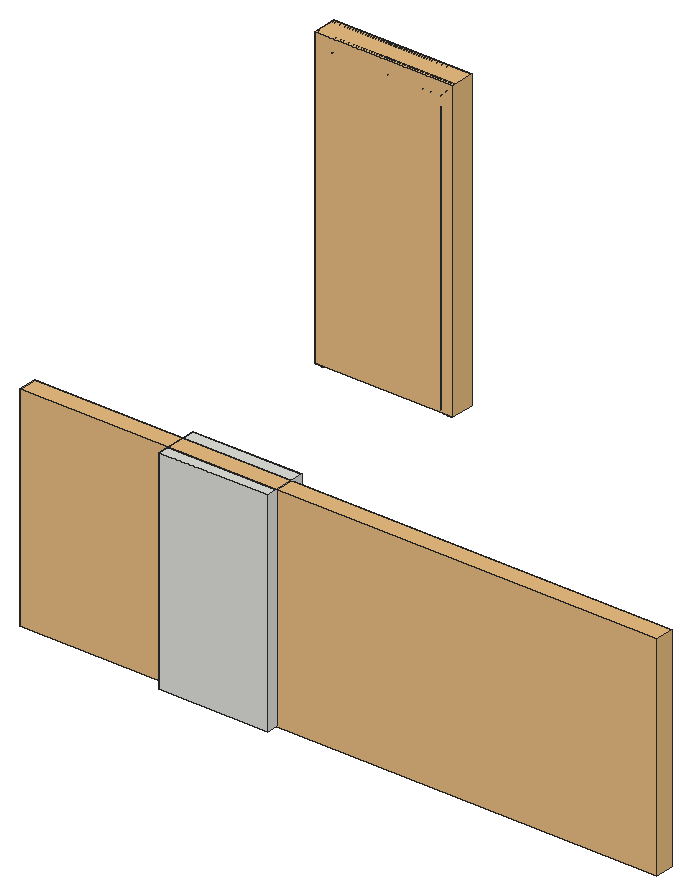
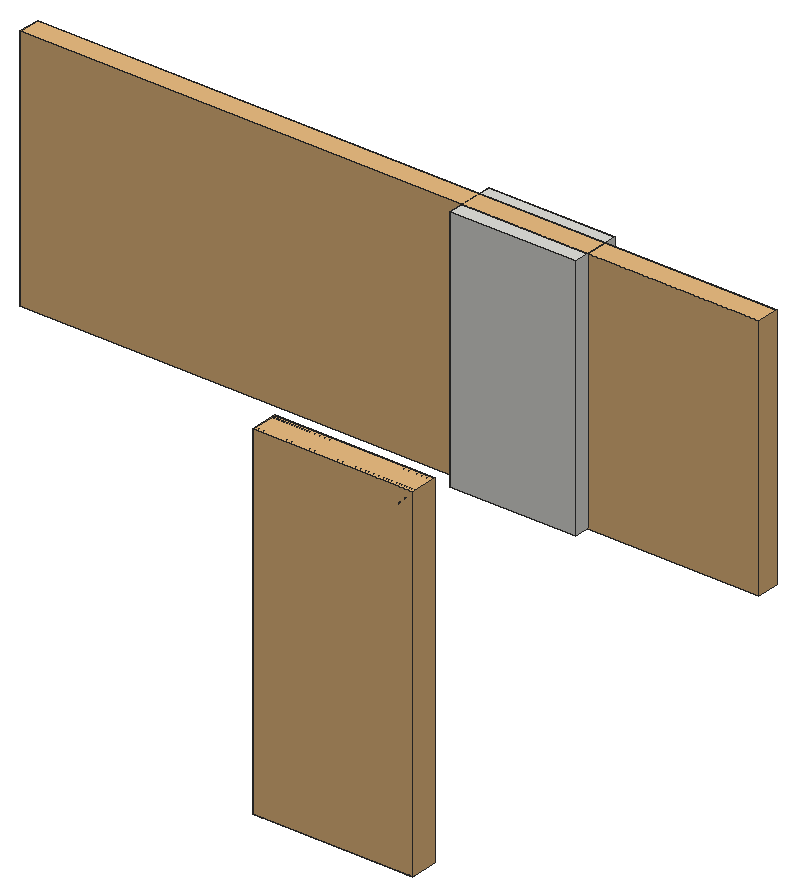
# SketchUp Ruby script. Lengths in inches.
U = 1.inch
M = Sketchup.active_model
def pt(a) = Geom::Point3d.new(a.map { |v| v * U })
def face(e, loops, mat)
  f = e.add_face(loops[0].map { |a| pt(a) })
  loops[1..].each { |l| e.add_face(l.map { |a| pt(a) }).erase! }
  f.material = f.back_material = mat if mat
  f
end
# faces: each face lists its corners as indices into pts; further lists are holes
def faces(e, pts, list, mat = nil) = list.each { |f| face(e, (f[0].is_a?(Array) ? f : [f]).map { |l| l.map { |i| pts[i] } }, mat) }
# xy, xz, yz: faces in a plane at the given z, y or x. An outline is a flat list of corners, or four numbers for a rectangle; further outlines are holes
def ring(l) = l.size == 4 ? [[l[0], l[1]], [l[2], l[1]], [l[2], l[3]], [l[0], l[3]]] : l.each_slice(2).to_a
def flat(e, list, mat, &to3) = list.each { |f| face(e, (f[0].is_a?(Array) ? f : [f]).map { |l| ring(l).map { |u, v| to3.(u, v) } }, mat) }
def xy(e, z, list, mat = nil) = flat(e, list, mat) { |x, y| [x, y, z] }
def xz(e, y, list, mat = nil) = flat(e, list, mat) { |x, z| [x, y, z] }
def yz(e, x, list, mat = nil) = flat(e, list, mat) { |y, z| [x, y, z] }
def lines(e, pts, list) = list.each { |a, b| e.add_line(pt(pts[a]), pt(pts[b])) }
# prism: a flat outline (further loops are holes) pulled along v
def prism(e, loops, v, mat = nil)
  f = face(e, loops, mat); d = Geom::Vector3d.new(v.map { |x| x * U })
  f.pushpull(f.normal.samedirection?(d) ? d.length : -d.length)
end
def box(e, o, s, mat = nil) = prism(e, [[o, [o[0] + s[0], o[1], o[2]], [o[0] + s[0], o[1] + s[1], o[2]], [o[0], o[1] + s[1], o[2]]]], [0, 0, s[2]], mat)
def at(x, y, z, deg = 0) = Geom::Transformation.translation(pt([x, y, z])) * Geom::Transformation.rotation(ORIGIN, Z_AXIS, deg.degrees)
def axes(o, x, y, z) = Geom::Transformation.new([*x, 0, *y, 0, *z, 0, *pt(o).to_a, 1])
def part(name) = M.definitions.add(name)
# library, detail: a bought-in or finely detailed component or shape, given as its bounding box
def library(name, o, s) = part(name).tap { |d| box(d.entities, o, s) }
def detail(e, o, s) = box(e.add_group.entities, o, s)
def put(e, d, t, mat = nil) = e.add_instance(d, t).tap { |i| i.material = mat if mat }
def group(e, t, mat = nil) = e.add_group.tap { |g| g.transformation = t; g.material = mat if mat }.entities
root = M.entities
M.materials.add("Material \#0").color = [86, 53, 35]
M.materials.add("Material \#1").color = [140, 140, 140]
c1 = library("Entrance gate assembly",[-0.09,68.76,-0.1],[180.01,5.32,60.06])
c2 = part("3DGeom~20_Defintion")
xy(c2.entities,0,[[-976.3,-241.71,-976.3,-223.46,23.7,-241.71],[23.7,-241.71,-976.3,-223.46,5.45,-223.46],[23.7,-241.71,5.45,-223.46,5.45,0],[23.7,-241.71,5.45,0,23.7,0],[-976.3,-223.46,-976.3,-211.85,5.45,-223.46],
  [5.45,-223.46,-976.3,-211.85,-6.16,-211.85],[5.45,-223.46,-6.16,-211.85,-6.16,0],[5.45,-223.46,-6.16,0,5.45,0],[-6.16,0,-6.16,211.85,5.45,223.46],[-6.16,0,5.45,223.46,5.45,0],
  [5.45,0,23.7,241.71,23.7,0],[5.45,0,5.45,223.46,23.7,241.71],[-976.3,211.85,-976.3,223.46,5.45,223.46],[-976.3,211.85,5.45,223.46,-6.16,211.85],[-976.3,223.46,-976.3,241.71,23.7,241.71],
  [-976.3,223.46,23.7,241.71,5.45,223.46]],"Material \#0")
c3 = part("3DGeom~18_Defintion")
xz(c3.entities,-241.71,[[-976.3,0,23.7,0,23.7,7.58],[-976.3,0,23.7,7.58,-976.3,7.58]],"Material \#0")
xz(c3.entities,241.71,[[-976.3,0,-976.3,7.58,23.7,7.58],[-976.3,0,23.7,7.58,23.7,0]],"Material \#0")
yz(c3.entities,23.7,[[-241.71,0,0,0,-241.71,7.58],[0,0,0,7.58,-241.71,7.58],[0,0,241.71,0,241.71,7.58],[0,0,241.71,7.58,0,7.58]],"Material \#0")
c4 = part("3DGeom~17_Defintion")
yz(c4.entities,-1908.8,[[-436.03,-21.87,-436.73,-21.5,-435.91,-21.83],[436.03,-21.87,435.91,-21.83,436.73,-21.5],[-435.91,-21.83,-436.73,-21.5,-436.15,-21.125],[-435.91,-21.83,-436.15,-21.125,-435.87,-21.72],[435.91,-21.83,435.87,-21.72,436.15,-21.125],
  [435.91,-21.83,436.15,-21.125,436.73,-21.5],[-436.73,-21.5,-484.73,-21.37,-436.15,-1.11],[-471.46,-21.5,-484.73,-21.37,-436.73,-21.5],[-477.2,-21.5,-484.73,-21.37,-471.46,-21.5],[-481.82,-21.5,-484.73,-21.37,-477.2,-21.5],
  [-436.73,-21.5,-436.15,-1.11,-436.15,-21.125],[436.73,-21.5,436.15,-21.125,471.46,-21.5],[471.46,-21.5,436.15,-21.125,477.2,-21.5],[477.2,-21.5,436.15,-21.125,499.98,-0.85],[477.2,-21.5,499.98,-0.85,481.82,-21.5],
  [481.82,-21.5,487.35,-21,484.73,-21.37],[481.82,-21.5,491.8,-19.52,487.35,-21],[481.82,-21.5,497.64,-13.67,491.8,-19.52],[481.82,-21.5,499.98,-0.85,497.64,-13.67],[-484.73,-21.37,-498.5,-11.58,-499.84,-0.37],
  [-484.73,-21.37,-499.84,-0.37,-499.4,-0.5],[-484.73,-21.37,-499.4,-0.5,-436.15,-1.11],[-484.73,-21.37,-493.63,-18.42,-498.5,-11.58],[-484.73,-21.37,-489.71,-20.375,-493.63,-18.42],[-484.73,-21.37,-487.35,-21,-489.71,-20.375],
  [436.15,-21.125,436.15,-1.11,436.73,-0.74],[436.15,-21.125,436.73,-0.74,499.98,-0.85],[487.35,-21,491.8,-19.52,489.71,-20.375],[-489.71,-20.375,-491.8,-19.52,-493.63,-18.42],[491.8,-19.52,495.21,-17.08,493.63,-18.42],
  [491.8,-19.52,497.64,-13.67,495.21,-17.08],[-493.63,-18.42,-496.54,-15.5,-498.5,-11.58],[-493.63,-18.42,-495.21,-17.08,-496.54,-15.5],[495.21,-17.08,497.64,-13.67,496.54,-15.5],[-496.54,-15.5,-497.64,-13.67,-498.5,-11.58],
  [497.64,-13.67,499.125,-9.22,498.5,-11.58],[497.64,-13.67,499.625,-3.69,499.125,-9.22],[497.64,-13.67,499.98,-0.85,499.625,-3.69],[-498.5,-11.58,-499.625,-3.69,-499.84,-0.37],[-498.5,-11.58,-499.5,-6.6,-499.625,-3.69],
  [-498.5,-11.58,-499.125,-9.22,-499.5,-6.6],[499.125,-9.22,499.625,-3.69,499.5,-6.6],[-499.625,-3.69,-499.98,-0.85,-500,-0.52],[-499.625,-3.69,-500,-0.52,-499.84,-0.37],[-436.15,-1.11,-499.4,-0.5,-471.46,-0.74],
  [-436.15,-1.11,-471.46,-0.74,-436.73,-0.74],[-436.15,-1.11,-436.73,-0.74,-435.91,-0.41],[-436.15,-1.11,-435.91,-0.41,-435.87,-0.52],[436.15,-1.11,435.87,-0.52,435.91,-0.41],[436.15,-1.11,435.91,-0.41,436.73,-0.74],
  [499.98,-0.85,436.73,-0.74,471.46,-0.74],[499.98,-0.85,471.46,-0.74,499.4,-0.5],[499.98,-0.85,499.4,-0.5,499.96,-0.41],[499.98,-0.85,499.96,-0.41,500,-0.52],[-436.73,-0.74,-436.03,-0.37,-435.91,-0.41],
  [436.73,-0.74,435.91,-0.41,436.03,-0.37],[-500,-0.52,-499.96,-0.41,-499.84,-0.37],[499.4,-0.5,499.84,-0.37,499.96,-0.41],[-499.84,141.21,-499.96,141.25,-499.4,141.35],[-436.03,141.21,-436.73,141.59,-435.91,141.25],
  [436.03,141.21,435.91,141.25,436.73,141.59],[499.84,141.21,484.73,162.21,498.5,152.42],[499.84,141.21,499.4,141.35,484.73,162.21],[499.84,141.21,498.5,152.42,499.625,144.53],[499.84,141.21,499.625,144.53,500,141.37],
  [499.84,141.21,500,141.37,499.96,141.25],[-499.96,141.25,-500,141.37,-499.98,141.69],[-499.96,141.25,-499.98,141.69,-499.4,141.35],[-435.91,141.25,-436.73,141.59,-436.15,141.96],[-435.91,141.25,-436.15,141.96,-435.87,141.37],
  [435.91,141.25,435.87,141.37,436.15,141.96],[435.91,141.25,436.15,141.96,436.73,141.59],[-499.4,141.35,-499.98,141.69,-471.46,141.59],[499.4,141.35,436.15,141.96,484.73,162.21],[499.4,141.35,471.46,141.59,436.15,141.96],
  [500,141.37,499.625,144.53,499.98,141.69],[-436.73,141.59,-499.98,141.69,-436.15,161.97],[-471.46,141.59,-499.98,141.69,-436.73,141.59],[-436.73,141.59,-436.15,161.97,-436.15,141.96],[436.73,141.59,436.15,141.96,471.46,141.59],
  [-499.98,141.69,-477.2,162.34,-436.15,161.97],[-499.98,141.69,-481.82,162.34,-477.2,162.34],[-499.98,141.69,-497.64,154.51,-481.82,162.34],[-499.98,141.69,-499.625,144.53,-497.64,154.51],[436.15,141.96,436.15,161.97,436.73,162.34],
  [436.15,141.96,436.73,162.34,484.73,162.21],[-499.625,144.53,-499.125,150.07,-497.64,154.51],[-499.625,144.53,-499.5,147.44,-499.125,150.07],[499.625,144.53,498.5,152.42,499.5,147.44],[499.5,147.44,498.5,152.42,499.125,150.07],
  [-499.125,150.07,-498.5,152.42,-497.64,154.51],[498.5,152.42,484.73,162.21,493.63,159.26],[498.5,152.42,493.63,159.26,496.54,156.34],[498.5,152.42,496.54,156.34,497.64,154.51],[-497.64,154.51,-491.8,160.36,-481.82,162.34],
  [-497.64,154.51,-495.21,157.92,-491.8,160.36],[-497.64,154.51,-496.54,156.34,-495.21,157.92],[496.54,156.34,493.63,159.26,495.21,157.92],[-495.21,157.92,-493.63,159.26,-491.8,160.36],[493.63,159.26,484.73,162.21,489.71,161.22],
  [493.63,159.26,489.71,161.22,491.8,160.36],[-491.8,160.36,-487.35,161.84,-481.82,162.34],[-491.8,160.36,-489.71,161.22,-487.35,161.84],[489.71,161.22,484.73,162.21,487.35,161.84],[-487.35,161.84,-484.73,162.21,-481.82,162.34],
  [-436.15,161.97,-477.2,162.34,-471.46,162.34],[-436.15,161.97,-471.46,162.34,-436.73,162.34],[-436.15,161.97,-436.73,162.34,-435.91,162.68],[-436.15,161.97,-435.91,162.68,-435.87,162.56],[436.15,161.97,435.87,162.56,435.91,162.68],
  [436.15,161.97,435.91,162.68,436.73,162.34],[484.73,162.21,436.73,162.34,471.46,162.34],[484.73,162.21,471.46,162.34,477.2,162.34],[484.73,162.21,477.2,162.34,481.82,162.34],[-436.73,162.34,-436.03,162.72,-435.91,162.68],
  [436.73,162.34,435.91,162.68,436.03,162.72]],"Material \#0")
c5 = library("3DGeom~16_Defintion",[-962.62,-252.34,-11.22],[1000,504.68,93.46])
c6 = part("3DGeom~22_Defintion")
xz(c6.entities,-210.625,[[-1016.13,2.47,-1016.13,9.96,-16.28,2.47],[-16.28,2.47,-1016.13,9.96,-16.28,9.96],[-1016.13,9.96,-1016.13,51.7,-16.28,51.7],[-1016.13,9.96,-16.28,51.7,-16.28,9.96],[-1016.13,51.7,-1016.13,72.71,-16.28,51.7]],"Material \#0")
xz(c6.entities,210.625,[[-1016.13,2.47,-16.28,2.47,-1016.13,9.96],[-16.28,2.47,-16.28,9.96,-1016.13,9.96],[-1016.13,9.96,-16.28,51.7,-1016.13,51.7],[-1016.13,9.96,-16.28,9.96,-16.28,51.7],[-1016.13,51.7,-16.28,51.7,-1016.13,72.71]],"Material \#0")
yz(c6.entities,-16.28,[[-210.625,2.47,-210.625,9.96,0,9.96],[-210.625,2.47,0,9.96,0,2.47],[0,2.47,0,9.96,210.625,2.47],[210.625,2.47,0,9.96,210.625,9.96],[-210.625,9.96,-210.625,51.7,0,51.7],
  [-210.625,9.96,0,51.7,0,9.96],[0,9.96,0,51.7,210.625,9.96],[210.625,9.96,0,51.7,210.625,51.7],[-210.625,51.7,0,72.71,0,51.7],[0,51.7,0,72.71,210.625,51.7]],"Material \#0")
p = [[-1016.13,-210.625,72.71],[-16.13,-210.77,73.09],[-16.28,-210.625,51.7],[-16.28,-210.625,51.7],[-16.13,-210.77,73.09],[-16.28,0,72.71],
  [-16.13,210.77,73.09],[-16.28,210.625,51.7],[-16.28,210.625,51.7],[-16.13,210.77,73.09],[-1016.13,210.625,72.71]]
faces(c6.entities,p,[[0,1,2],[3,4,5],[5,6,7],[8,9,10]],"Material \#0")
c7 = part("3DGeom~15_Defintion")
xy(c7.entities,0,[[-961.58,-251.9,-958.5,-248.8125,-961.58,-237.8],[-961.58,-251.9,28.8,-248.8125,-958.5,-248.8125],[-961.58,-251.9,36.25,-251.9,28.8,-248.8125],[36.25,-251.9,19.98,-239.99,28.8,-248.8125],[36.25,-251.9,22.16,-237.8,19.98,-239.99],
  [-958.5,-248.8125,-958.5,-237.8,-961.58,-237.8],[19.98,-239.99,22.16,-237.8,3.36,-223.37],[-958.5,-237.8,-958.5,-223.37,-961.58,-220.28],[-961.58,-237.8,-958.5,-237.8,-961.58,-220.28],[22.16,-237.8,4.64,-220.28,3.36,-223.37],
  [-958.5,-223.37,4.64,-220.28,-961.58,-220.28],[-958.5,-223.37,3.36,-223.37,4.64,-220.28],[5.29,-219.63,8.375,-218.35,5.29,0],[8.375,-218.35,8.375,0,5.29,0],[5.29,0,8.375,0,5.29,219.63],
  [8.375,0,8.375,218.35,5.29,219.63],[8.375,218.35,22.8125,237.15,5.29,219.63],[-961.58,220.28,-958.5,223.37,-961.58,237.8],[-961.58,220.28,3.36,223.37,-958.5,223.37],[-961.58,220.28,4.64,220.28,3.36,223.37],
  [4.64,220.28,19.98,239.99,3.36,223.37],[4.64,220.28,22.16,237.8,19.98,239.99],[-958.5,223.37,-958.5,237.8,-961.58,237.8],[-958.5,237.8,-958.5,248.8125,-961.58,251.9],[-961.58,237.8,-958.5,237.8,-961.58,251.9],
  [22.16,237.8,28.8,248.8125,19.98,239.99],[22.16,237.8,36.25,251.9,28.8,248.8125],[-958.5,248.8125,36.25,251.9,-961.58,251.9],[-958.5,248.8125,28.8,248.8125,36.25,251.9]],"Material \#0")
xy(c7.entities,7.48,[[-962.79,-238.36,23.37,-238.36,-962.79,-219.67],[23.37,-238.36,4.67,-219.67,-962.79,-219.67],[23.37,-238.36,23.37,0,4.67,-219.67],[4.67,-219.67,23.37,0,4.67,0],[23.37,0,23.37,238.36,4.67,219.67],
  [4.67,0,23.37,0,4.67,219.67],[-962.79,219.67,23.37,238.36,-962.79,238.36],[-962.79,219.67,4.67,219.67,23.37,238.36]],"Material \#0")
xy(c7.entities,63.5625,[[-962.79,-238.36,-962.79,-219.67,4.67,-219.67],[-962.79,-238.36,4.67,-219.67,23.37,-238.36],[23.37,-238.36,4.67,-219.67,23.37,0],[4.67,-219.67,4.67,0,23.37,0],[23.37,0,4.67,219.67,23.37,238.36],
  [4.67,0,4.67,219.67,23.37,0],[-962.79,219.67,-962.79,238.36,4.67,219.67],[4.67,219.67,-962.79,238.36,23.37,238.36]],"Material \#0")
xy(c7.entities,69.64,[[-962.79,-219.62,4.63,-219.62,-962.79,-200.32],[4.63,-219.62,-14.68,-200.32,-962.79,-200.32],[4.63,-219.62,4.63,0,-14.68,-200.32],[-14.68,-200.32,4.63,0,-14.68,0],[-14.68,0,4.63,0,-14.68,200.32],
  [4.63,0,4.63,219.62,-14.68,200.32],[-962.79,200.32,-14.68,200.32,4.63,219.62],[-962.79,200.32,4.63,219.62,-962.79,219.62]],"Material \#0")
xy(c7.entities,71.04,[[-961.58,-251.9,-958.5,-248.8125,28.8,-248.8125],[-961.58,-251.9,-961.58,-237.8,-958.5,-248.8125],[-961.58,-251.9,28.8,-248.8125,36.25,-251.9],[36.25,-251.9,19.98,-239.99,22.16,-237.8],[36.25,-251.9,28.8,-248.8125,19.98,-239.99],
  [-958.5,-248.8125,-961.58,-237.8,-958.5,-237.8],[19.98,-239.99,3.36,-223.37,22.16,-237.8],[-958.5,-237.8,-961.58,-220.28,-958.5,-223.37],[-961.58,-237.8,-961.58,-220.28,-958.5,-237.8],[22.16,-237.8,3.36,-223.37,4.64,-220.28],
  [-958.5,-223.37,-961.58,-220.28,4.64,-220.28],[-958.5,-223.37,4.64,-220.28,3.36,-223.37],[5.29,-219.63,5.29,0,8.375,-218.35],[8.375,-218.35,5.29,0,8.375,0],[5.29,0,5.29,219.63,8.375,0],
  [8.375,0,5.29,219.63,8.375,218.35],[8.375,218.35,5.29,219.63,22.8125,237.15],[-961.58,220.28,-958.5,223.37,3.36,223.37],[-961.58,220.28,-961.58,237.8,-958.5,223.37],[-961.58,220.28,3.36,223.37,4.64,220.28],
  [4.64,220.28,3.36,223.37,19.98,239.99],[4.64,220.28,19.98,239.99,22.16,237.8],[-958.5,223.37,-961.58,237.8,-958.5,237.8],[-958.5,237.8,-961.58,251.9,-958.5,248.8125],[-961.58,237.8,-961.58,251.9,-958.5,237.8],
  [22.16,237.8,19.98,239.99,28.8,248.8125],[22.16,237.8,28.8,248.8125,36.25,251.9],[-958.5,248.8125,-961.58,251.9,36.25,251.9],[-958.5,248.8125,36.25,251.9,28.8,248.8125]],"Material \#0")
xz(c7.entities,-238.36,[[-962.79,63.5625,23.37,63.5625,23.37,72.07],[-962.79,63.5625,23.37,72.07,-962.79,72.07]],"Material \#0")
xz(c7.entities,-219.67,[[-962.79,7.48,4.67,7.48,-962.79,63.5625],[4.67,7.48,4.67,63.5625,-962.79,63.5625]],"Material \#0")
xz(c7.entities,219.67,[[-962.79,7.48,-962.79,63.5625,4.67,7.48],[4.67,7.48,-962.79,63.5625,4.67,63.5625]],"Material \#0")
xz(c7.entities,238.36,[[-962.79,63.5625,-962.79,72.07,23.37,72.07],[-962.79,63.5625,23.37,72.07,23.37,63.5625]],"Material \#0")
yz(c7.entities,4.67,[[-219.67,7.48,0,7.48,-219.67,63.5625],[0,7.48,0,63.5625,-219.67,63.5625],[0,7.48,219.67,63.5625,0,63.5625],[0,7.48,219.67,7.48,219.67,63.5625]],"Material \#0")
yz(c7.entities,23.37,[[-238.36,63.5625,0,63.5625,-238.36,72.07],[0,63.5625,0,72.07,-238.36,72.07],[0,63.5625,238.36,63.5625,238.36,72.07],[0,63.5625,238.36,72.07,0,72.07]],"Material \#0")
p = [[36.9,-251.24,0],[37.21,0,-0.16],[34.125,0,-0.14],[36.9,251.24,0],[33.83,243.81,0.02],[33.83,-243.8,0.02],
  [22.8125,-237.15,0],[24.99,-234.97,-0.01],[5.375,-220.37,0],[23.37,-238.36,7.48],[4.67,-219.67,7.48],[4.67,-219.67,7.48],
  [23.37,-238.36,7.48],[23.37,-238.36,0],[4.67,-219.67,7.48],[23.37,-238.36,0],[5.375,-220.37,0],[5.375,-220.37,0],
  [23.37,-238.36,0],[5.29,-219.63,0],[8.375,-218.35,0],[-15.36,-199.64,1.62],[4.67,-219.67,7.48],[5.375,-220.37,0],
  [-13.8,-201.19,0.06],[5.375,-220.37,0],[5.375,-220.37,0],[-14.84,-200.15,0.58],[5.375,-220.37,0],[-13.8,-201.19,0.06],
  [-6.08,-208.92,0],[5.375,-220.37,0],[-13.8,-201.19,0.06],[-6.08,-208.92,0],[-13.8,-201.19,0.06],[5.375,-220.37,0],
  [-6.08,-208.92,0],[-13.8,-201.19,0.06],[-13.09,-201.91,0],[-6.08,-208.92,0],[-13.09,-201.91,0],[-13.8,-201.19,0.06],
  [-15.36,199.64,1.62],[4.67,219.67,7.48],[5.375,220.37,0],[-13.8,201.19,0.06],[5.375,220.37,0],[5.375,220.37,0],
  [4.67,219.67,7.48],[-14.84,200.15,0.58],[5.375,220.37,0],[-13.8,201.19,0.06],[-6.08,208.92,0],[-13.09,201.91,0],
  [-13.8,201.19,0.06],[-6.08,208.92,0],[-13.8,201.19,0.06],[5.375,220.37,0],[-6.08,208.92,0],[5.375,220.37,0],
  [-13.8,201.19,0.06],[-6.08,208.92,0],[-13.8,201.19,0.06],[-13.09,201.91,0],[8.375,218.35,0],[24.99,234.97,-0.01],
  [22.8125,237.15,0],[23.37,238.36,7.48],[23.37,238.36,0],[23.37,238.36,0],[5.375,220.37,0],[5.375,220.37,0],
  [23.37,238.36,7.48],[4.67,219.67,7.48],[5.375,220.37,0],[23.37,238.36,0],[23.37,238.36,7.48],[-13.8,-201.19,0.06],
  [-14.84,-200.15,0.58],[-14.38,-200.61,0.26],[-13.8,-201.19,0.06],[-13.8,-201.19,0.06],[-14.38,-200.61,0.26],[-13.8,201.19,0.06],
  [-14.84,200.15,0.58],[-13.8,201.19,0.06],[-14.38,200.61,0.26],[-14.38,200.61,0.26],[-13.8,201.19,0.06],[4.63,-219.62,69.64],
  [4.63,-219.62,69.64],[-15.42,-199.57,9.43],[-15.36,-199.64,1.62],[-15.16,-199.83,1.04],[-15.16,-199.83,1.04],[-15.16,199.83,1.04],
  [-15.36,199.64,1.62],[-15.16,199.83,1.04],[-15.42,199.57,9.43],[4.63,219.62,69.64],[4.67,219.67,7.48],[4.63,219.62,69.64],
  [4.63,-219.62,69.64],[4.67,-219.67,63.5625],[4.67,-219.67,63.5625],[4.67,-219.67,7.48],[-15.28,-199.71,69.25],[4.63,-219.62,69.64],
  [-15.42,-199.57,9.43],[-15.28,-199.71,69.25],[-15.42,-199.57,2.34],[-15.42,-199.57,2.34],[-15.42,199.57,2.34],[-15.42,199.57,9.43],
  [-15.28,199.71,69.25],[-15.28,199.71,69.25],[4.63,219.62,69.64],[4.63,219.62,69.64],[4.67,219.67,63.5625],[4.67,219.67,63.5625],
  [-15.42,199.57,2.34],[4.67,-219.67,63.5625],[4.63,-219.62,69.64],[4.67,219.67,7.48],[4.67,219.67,63.5625],[4.63,219.62,69.64],
  [4.63,-219.62,69.64],[-15.28,-199.71,69.25],[-15.28,-199.71,69.25],[-15.42,-199.57,48.99],[-15.42,-199.57,48.99],[-15.28,-199.71,69.25],
  [-15.42,199.57,48.99],[-15.28,199.71,69.25],[-15.28,199.71,69.25],[-15.42,199.57,48.99],[4.63,219.62,69.64],[4.63,-219.62,69.64],
  [23.37,-238.36,72.07],[4.67,-219.67,63.5625],[4.67,-219.67,63.5625],[23.37,-238.36,63.5625],[23.37,-238.36,72.07],[4.67,-219.67,63.5625],
  [5.24,-220.23,70.03],[23.37,-238.36,72.07],[23.37,-238.36,63.5625],[4.67,-219.67,63.5625],[4.67,-219.67,63.5625],[4.63,-219.62,69.64],
  [4.63,219.62,69.64],[23.37,238.36,72.07],[4.67,219.67,63.5625],[4.67,219.67,63.5625],[5.24,220.23,70.03],[4.63,219.62,69.64],
  [23.37,238.36,63.5625],[4.67,219.67,63.5625],[4.67,219.67,63.5625],[23.37,238.36,63.5625],[23.37,238.36,72.07],[4.67,219.67,63.5625],
  [23.37,238.36,72.07],[4.63,-219.62,69.64],[-14.68,-200.32,69.64],[-15.28,-199.71,69.25],[-15.28,-199.71,69.25],[-14.68,-200.32,69.64],
  [4.63,-219.62,69.64],[-15.28,199.71,69.25],[-14.68,200.32,69.64],[4.63,219.62,69.64],[4.63,219.62,69.64],[-14.68,200.32,69.64],
  [4.63,-219.62,69.64],[5.24,-220.23,70.03],[23.37,-238.36,72.07],[4.63,219.62,69.64],[5.24,220.23,70.03],[5.375,-220.37,72.07],
  [5.375,-220.37,72.07],[23.37,-238.36,72.07],[5.375,220.37,72.07],[23.37,238.36,72.07],[5.375,220.37,72.07],[33.83,-243.8,71.03],
  [36.9,-251.24,71.04],[22.8125,-237.15,71.04],[34.125,0,71.19],[37.21,0,71.2],[24.99,-234.97,71.05],[5.29,-219.63,71.04],
  [8.375,-218.35,71.04],[33.83,243.81,71.03],[36.9,251.24,71.04],[22.8125,237.15,71.04],[24.99,234.97,71.05],[8.375,218.35,71.04]]
faces(c7.entities,p,[[0,1,2],[1,3,4],[4,2,1],[2,5,0],[6,0,5],[5,7,6],[8,9,10],[11,12,13],
  [14,15,16],[17,18,9],[19,6,7],[7,20,19],[21,22,23],[24,21,25],[26,10,27],[28,27,29],
  [30,31,32],[33,34,35],[36,37,38],[39,40,41],[42,43,44],[45,42,46],[47,48,49],[50,49,51],
  [52,53,54],[55,56,57],[58,59,60],[61,62,63],[64,65,66],[43,67,68],[43,69,70],[71,72,73],
  [74,75,76],[3,66,65],[65,4,3],[77,78,21],[27,79,80],[81,82,78],[83,84,42],[85,86,84],
  [49,87,88],[10,89,27],[90,91,27],[92,93,27],[91,92,27],[78,94,21],[84,95,42],[96,97,49],
  [98,96,49],[99,98,49],[100,101,49],[21,102,103],[21,104,105],[21,106,107],[21,108,109],[91,110,92],
  [21,111,108],[42,112,113],[42,113,114],[42,115,116],[42,117,118],[42,119,43],[98,120,96],[10,121,122],
  [123,124,125],[126,127,91],[128,129,91],[108,130,131],[113,132,133],[134,135,98],[136,134,98],[137,138,139],
  [140,141,142],[143,142,144],[145,146,147],[148,144,149],[150,151,152],[153,154,155],[151,156,157],[158,159,160],
  [161,162,154],[163,164,165],[166,167,168],[169,170,171],[172,173,134],[174,175,176],[177,178,151],[142,179,144],
  [175,180,181],[178,182,151],[183,184,154],[185,186,187],[186,185,188],[188,189,186],[187,190,185],[190,187,191],
  [191,192,190],[189,188,193],[193,194,189],[195,196,197],[196,195,194],[194,193,196]],"Material \#0")
c8 = part("3DGeom~19_Defintion")
xy(c8.entities,0,[[-6.28,-215.79,-994.45,-208.55,-13.52,-208.55],[-994.45,-215.79,-994.45,-208.55,-6.28,-215.79],[-6.28,-215.79,-13.52,-208.55,-13.52,0],[-6.28,-215.79,-13.52,0,-6.28,0],[-13.52,0,-13.52,208.55,-6.28,215.79],
  [-13.52,0,-6.28,215.79,-6.28,0],[-994.45,208.55,-6.28,215.79,-13.52,208.55],[-994.45,208.55,-994.45,215.79,-6.28,215.79]],"Material \#0")
p = [[-13.52,-208.55,0],[-994.45,-208.55,0],[-994.45,-207.81,0.07],[-14.25,-207.81,0.07],[-13.52,-208.55,0],[-14.25,-207.81,0.07],
  [-14.25,0,0.07],[-13.52,0,0],[-13.52,208.55,0],[-14.25,207.81,0.07],[-13.52,208.55,0],[-14.25,207.81,0.07],
  [-994.45,207.81,0.07],[-994.45,208.55,0],[-994.45,-207.21,0.27],[-994.45,-207.21,0.27],[-14.86,-207.21,0.27],[-14.86,-207.21,0.27],
  [-14.86,0,0.27],[-14.86,0,0.27],[-14.86,0,0.27],[-14.86,0,0.27],[-14.86,207.21,0.27],[-14.86,207.21,0.27],
  [-994.45,207.21,0.27],[-994.45,207.21,0.27],[-14.86,-207.21,0.27],[-994.45,-207.21,0.27],[-994.45,-206.74,0.6],[-15.33,-206.74,0.6],
  [-14.86,-207.21,0.27],[-15.33,-206.74,0.6],[-15.33,0,0.6],[-14.86,0,0.27],[-14.86,207.21,0.27],[-15.33,206.74,0.6],
  [-14.86,207.21,0.27],[-15.33,206.74,0.6],[-994.45,206.74,0.6],[-994.45,207.21,0.27],[-994.45,-206.4,1.07],[-15.66,-206.4,1.07],
  [-15.66,-206.4,1.07],[-15.66,0,1.07],[-15.66,206.4,1.07],[-15.66,206.4,1.07],[-994.45,206.4,1.07],[-994.45,-206.2,1.68],
  [-15.86,-206.2,1.68],[-15.86,-206.2,1.68],[-15.86,0,1.68],[-15.86,206.2,1.68],[-15.86,206.2,1.68],[-994.45,206.2,1.68],
  [-994.45,-206.13,2.41],[-15.93,-206.13,2.41],[-15.93,-206.13,2.41],[-15.93,0,2.41],[-15.93,206.13,2.41],[-15.93,206.13,2.41],
  [-994.45,206.13,2.41],[-994.45,-206.13,71.16],[-994.45,-206.22,71.59],[-15.79,-206.28,71.53],[-15.79,-206.28,71.53],[-15.84,0,71.59],
  [-15.93,0,71.16],[-15.79,206.28,71.53],[-15.79,206.28,71.53],[-994.45,206.22,71.59],[-994.45,206.13,71.16],[-15.79,-206.28,71.53],
  [-994.45,-206.48,71.84],[-994.45,-206.9,71.93],[-15.16,-206.9,71.93],[-15.79,-206.28,71.53],[-15.79,-206.28,71.53],[-15.16,-206.9,71.93],
  [-15.16,0,71.93],[-994.45,-206.48,71.84],[-15.59,0,71.84],[-15.79,-206.28,71.53],[-15.59,0,71.84],[-15.79,206.28,71.53],
  [-15.16,206.9,71.93],[-15.59,0,71.84],[-15.79,206.28,71.53],[-994.45,206.48,71.84],[-15.79,206.28,71.53],[-15.16,206.9,71.93],
  [-994.45,206.9,71.93],[-994.45,206.48,71.84],[-15.79,206.28,71.53],[-994.45,-227.27,72.01],[5.41,-227.47,72.33],[4.78,-226.84,71.93],
  [4.78,-226.84,71.93],[5.41,-227.47,72.33],[5.21,0,72.01],[-994.45,-226.84,71.93],[-994.45,-227.27,72.01],[5.21,0,72.01],
  [4.78,0,71.93],[4.78,226.84,71.93],[5.21,0,72.01],[5.21,0,72.01],[5.41,227.47,72.33],[4.78,226.84,71.93],
  [5.41,227.47,72.33],[-994.45,227.27,72.01],[-994.45,227.27,72.01],[-994.45,226.84,71.93],[-994.45,-227.27,72.01],[-994.45,-227.53,72.27],
  [5.41,-227.47,72.33],[5.41,-227.47,72.33],[5.47,0,72.27],[5.21,0,72.01],[5.41,227.47,72.33],[5.41,227.47,72.33],
  [-994.45,227.53,72.27],[-994.45,227.27,72.01],[-994.45,-227.61,72.7],[-994.45,-227.61,74.4375],[-994.45,-227.61,74.4375],[5.55,-227.61,74.4375],
  [5.55,-227.61,74.4375],[5.55,0,74.4375],[5.55,0,72.7],[5.55,227.61,74.4375],[5.55,227.61,74.4375],[-994.45,227.61,74.4375],
  [-994.45,227.61,74.4375],[-994.45,227.61,72.7]]
faces(c8.entities,p,[[0,1,2],[2,3,0],[4,5,6],[6,7,4],[8,7,6],[6,9,8],[10,11,12],[12,13,10],
  [3,2,14],[15,16,3],[5,17,18],[19,6,5],[9,6,20],[21,22,9],[11,23,24],[25,12,11],
  [26,27,28],[28,29,26],[30,31,32],[32,33,30],[34,33,32],[32,35,34],[36,37,38],[38,39,36],
  [29,28,40],[40,41,29],[31,42,43],[43,32,31],[35,32,43],[43,44,35],[37,45,46],[46,38,37],
  [41,40,47],[47,48,41],[42,49,50],[50,43,42],[44,43,50],[50,51,44],[45,52,53],[53,46,45],
  [48,47,54],[54,55,48],[49,56,57],[57,50,49],[51,50,57],[57,58,51],[52,59,60],[60,53,52],
  [61,62,63],[64,65,66],[66,65,67],[68,69,70],[71,72,73],[73,74,75],[76,77,78],[62,79,63],
  [78,80,76],[81,82,65],[83,80,78],[78,84,83],[65,85,86],[68,87,69],[88,89,90],[90,91,92],
  [93,94,95],[96,97,98],[95,99,100],[101,102,96],[103,102,104],[105,106,103],[107,108,109],[110,111,107],
  [112,113,114],[115,116,117],[117,116,118],[119,120,121],[114,122,123],[124,125,114],[113,122,114],[115,126,127],
  [127,128,115],[115,128,116],[118,128,127],[127,129,118],[116,128,118],[119,130,131],[132,133,119],[119,133,120]],"Material \#0")
box(root,[164.741,60,0],[30.738,12,60])
xz(root,196.69,[[109.188,40.472,109.188,40.48,109.138,40.479],[109.188,40.472,109.236,40.487,109.188,40.48],[109.188,40.472,109.238,40.479,109.236,40.487],[109.138,40.479,109.14,40.487,109.092,40.5],[109.138,40.479,109.188,40.48,109.14,40.487],
  [109.238,40.479,109.281,40.507,109.236,40.487],[109.238,40.479,109.285,40.5,109.281,40.507],[109.14,40.487,109.095,40.507,109.092,40.5],[109.092,40.5,109.095,40.507,109.052,40.534],[109.285,40.5,109.319,40.539,109.281,40.507],
  [109.285,40.5,109.325,40.534,109.319,40.539],[109.095,40.507,109.057,40.539,109.052,40.534],[109.052,40.534,109.057,40.539,109.021,40.577],[109.325,40.534,109.349,40.581,109.319,40.539],[109.325,40.534,109.355,40.577,109.349,40.581],
  [109.057,40.539,109.027,40.581,109.021,40.577],[109.021,40.577,109.027,40.581,109.002,40.628],[109.355,40.577,109.368,40.63,109.349,40.581],[109.355,40.577,109.375,40.628,109.368,40.63],[109.027,40.581,109.009,40.63,109.002,40.628],
  [109.002,40.628,109.009,40.63,108.995,40.682],[109.375,40.628,109.374,40.682,109.368,40.63],[109.375,40.628,109.381,40.682,109.374,40.682],[109.009,40.63,109.002,40.682,108.995,40.682],[108.995,40.682,109.002,40.682,109.002,40.737],
  [109.002,40.682,109.009,40.735,109.002,40.737],[109.374,40.682,109.381,40.682,109.368,40.735],[109.381,40.682,109.375,40.737,109.368,40.735],[109.009,40.735,109.021,40.787,109.002,40.737],[109.009,40.735,109.027,40.783,109.021,40.787],
  [109.368,40.735,109.375,40.737,109.349,40.783],[109.375,40.737,109.355,40.787,109.349,40.783],[109.027,40.783,109.052,40.831,109.021,40.787],[109.027,40.783,109.057,40.825,109.052,40.831],[109.349,40.783,109.355,40.787,109.319,40.825],
  [109.355,40.787,109.325,40.831,109.319,40.825],[109.057,40.825,109.092,40.864,109.052,40.831],[109.057,40.825,109.095,40.857,109.092,40.864],[109.319,40.825,109.325,40.831,109.281,40.857],[109.325,40.831,109.285,40.864,109.281,40.857],
  [109.095,40.857,109.138,40.885,109.092,40.864],[109.095,40.857,109.14,40.877,109.138,40.885],[109.281,40.857,109.285,40.864,109.236,40.877],[109.285,40.864,109.238,40.885,109.236,40.877],[109.14,40.877,109.188,40.892,109.138,40.885],
  [109.14,40.877,109.188,40.884,109.188,40.892],[109.236,40.877,109.238,40.885,109.188,40.884],[109.188,40.884,109.238,40.885,109.188,40.892]],"Material \#1")
xz(root,196.7,[[109.188,40.003,109.295,40.059,109.081,40.059],[109.188,40.003,109.22,40.007,109.248,40.018],[109.188,40.003,109.248,40.018,109.295,40.059],[109.248,40.018,109.274,40.036,109.295,40.059],[109.295,40.059,109.188,40.447,109.138,40.453],
  [109.295,40.059,109.325,40.152,109.188,40.447],[109.295,40.059,109.311,40.087,109.322,40.118],[109.295,40.059,109.322,40.118,109.325,40.152],[109.325,40.152,109.238,40.453,109.188,40.447],[109.325,40.152,109.283,40.471,109.238,40.453],
  [109.325,40.152,109.324,40.498,109.283,40.471],[109.325,40.152,109.325,40.4375,109.324,40.498],[109.325,40.4375,109.327,40.45,109.324,40.498],[109.325,40.4375,109.326,40.444,109.327,40.45],[109.327,40.45,109.357,40.535,109.324,40.498],
  [109.327,40.45,109.328,40.456,109.331,40.461],[109.327,40.45,109.331,40.461,109.357,40.535],[109.331,40.461,109.334,40.466,109.431,40.647],[109.331,40.461,109.383,40.579,109.357,40.535],[109.331,40.461,109.431,40.647,109.383,40.579],
  [109.334,40.466,109.338,40.47,109.431,40.647],[109.338,40.47,109.342,40.475,109.384,40.524],[109.338,40.47,109.384,40.524,109.431,40.647],[109.342,40.475,109.364,40.498,109.384,40.524],[109.384,40.524,109.401,40.551,109.415,40.581],
  [109.384,40.524,109.415,40.581,109.431,40.647],[109.383,40.579,109.431,40.647,109.399,40.628],[109.415,40.581,109.425,40.613,109.431,40.647],[109.399,40.628,109.431,40.647,109.405,40.682],[109.431,40.647,109.38,40.849,109.383,40.786],
  [109.431,40.647,109.427,40.743,109.38,40.849],[109.431,40.647,109.383,40.786,109.399,40.736],[109.431,40.647,109.399,40.736,109.405,40.682],[109.431,40.647,109.434,40.682,109.427,40.743],[109.427,40.743,109.409,40.8,109.38,40.849],
  [109.383,40.786,109.38,40.849,109.357,40.829],[109.357,40.829,109.38,40.849,109.324,40.866],[109.38,40.849,109.188,40.949,109.283,40.894],[109.38,40.849,109.296,40.922,109.188,40.949],[109.38,40.849,109.283,40.894,109.324,40.866],
  [109.38,40.849,109.342,40.89,109.296,40.922],[109.283,40.894,109.188,40.949,109.238,40.912],[109.238,40.912,109.188,40.949,109.188,40.918],[109.296,40.922,109.244,40.942,109.188,40.949]],"Material \#1")
xz(root,196.734,[[109.188,37.641,109.3,37.663,109.188,37.652],[109.188,37.641,109.302,37.652,109.3,37.663],[109.302,37.652,109.405,37.695,109.3,37.663],[109.302,37.652,109.408,37.684,109.405,37.695],[109.408,37.684,109.501,37.745,109.405,37.695],
  [109.408,37.684,109.507,37.734,109.501,37.745],[109.507,37.734,109.588,37.811,109.501,37.745],[109.507,37.734,109.595,37.802,109.588,37.811],[109.595,37.802,109.663,37.893,109.588,37.811],[109.595,37.802,109.671,37.885,109.663,37.893],
  [109.188,37.824,109.224,37.84,109.188,37.836],[109.188,37.824,109.226,37.828,109.224,37.84],[109.226,37.828,109.257,37.85,109.224,37.84],[109.226,37.828,109.261,37.839,109.257,37.85],[109.261,37.839,109.288,37.866,109.257,37.85],
  [109.261,37.839,109.294,37.855,109.288,37.866],[109.294,37.855,109.316,37.887,109.288,37.866],[109.294,37.855,109.323,37.878,109.316,37.887],[109.323,37.878,109.34,37.913,109.316,37.887],[109.323,37.878,109.348,37.905,109.34,37.913],
  [109.671,37.885,109.724,37.987,109.663,37.893],[109.671,37.885,109.733,37.981,109.724,37.987],[109.348,37.905,109.36,37.943,109.34,37.913],[109.348,37.905,109.369,37.937,109.36,37.943],[109.369,37.937,109.375,37.977,109.36,37.943],
  [109.369,37.937,109.385,37.973,109.375,37.977],[109.385,37.973,109.384,38.014,109.375,37.977],[109.385,37.973,109.395,38.012,109.384,38.014],[109.733,37.981,109.77,38.092,109.724,37.987],[109.733,37.981,109.78,38.088,109.77,38.092],
  [109.395,38.012,109.387,38.052,109.384,38.014],[109.395,38.012,109.398,38.052,109.387,38.052],[109.387,38.052,109.398,38.052,109.384,38.091],[109.398,38.052,109.395,38.093,109.384,38.091],[109.78,38.088,109.799,38.206,109.77,38.092],
  [109.78,38.088,109.809,38.204,109.799,38.206],[109.384,38.091,109.395,38.093,109.375,38.128],[109.395,38.093,109.385,38.132,109.375,38.128],[109.375,38.128,109.385,38.132,109.36,38.161],[109.385,38.132,109.369,38.167,109.36,38.161],
  [109.36,38.161,109.369,38.167,109.34,38.192],[109.369,38.167,109.348,38.199,109.34,38.192],[109.34,38.192,109.348,38.199,109.316,38.218],[109.348,38.199,109.323,38.227,109.316,38.218],[109.809,38.204,109.809,38.332,109.799,38.206],
  [109.809,38.204,109.82,38.331,109.809,38.332],[109.316,38.218,109.323,38.227,109.288,38.239],[109.323,38.227,109.294,38.249,109.288,38.239],[109.288,38.239,109.294,38.249,109.257,38.255],[109.294,38.249,109.261,38.266,109.257,38.255],
  [109.257,38.255,109.261,38.266,109.224,38.265],[109.224,38.265,109.226,38.277,109.188,38.269],[109.224,38.265,109.261,38.266,109.226,38.277],[109.188,38.269,109.226,38.277,109.188,38.28],[109.82,38.331,109.809,44.483,109.809,38.332]],"Material \#1")
put(root,c1,at(302.91,137.08,0.1,180))
put(root,c2,axes([122.55,192.81,83.86],[0,0,0.08282],[0.07619,0,0],[0,0.07084,0]),"Material \#0")
put(root,c3,axes([122.55,192.81,83.86],[0,0,0.08282],[0.07619,0,0],[0,0.07084,0]),"Material \#0")
put(root,c4,axes([122.55,192.81,83.86],[0,0,0.04236],[0.03897,0,0],[0,0.03623,0]),"Material \#0")
put(root,c5,axes([122.55,192.81,83.86],[0,0,0.084],[0.07728,0,0],[0,0.07184,0]),"Material \#0")
put(root,c6,axes([122.55,192.81,83.86],[0,0,0.07958],[0.07321,0,0],[0,0.06806,0]),"Material \#0")
put(root,c7,axes([122.55,192.81,83.86],[0,0,0.08398],[0.07726,0,0],[0,0.07183,0]),"Material \#0")
put(root,c8,axes([122.55,192.81,83.86],[0,0,0.08131],[0.0748,0,0],[0,0.06954,0]),"Material \#0")
